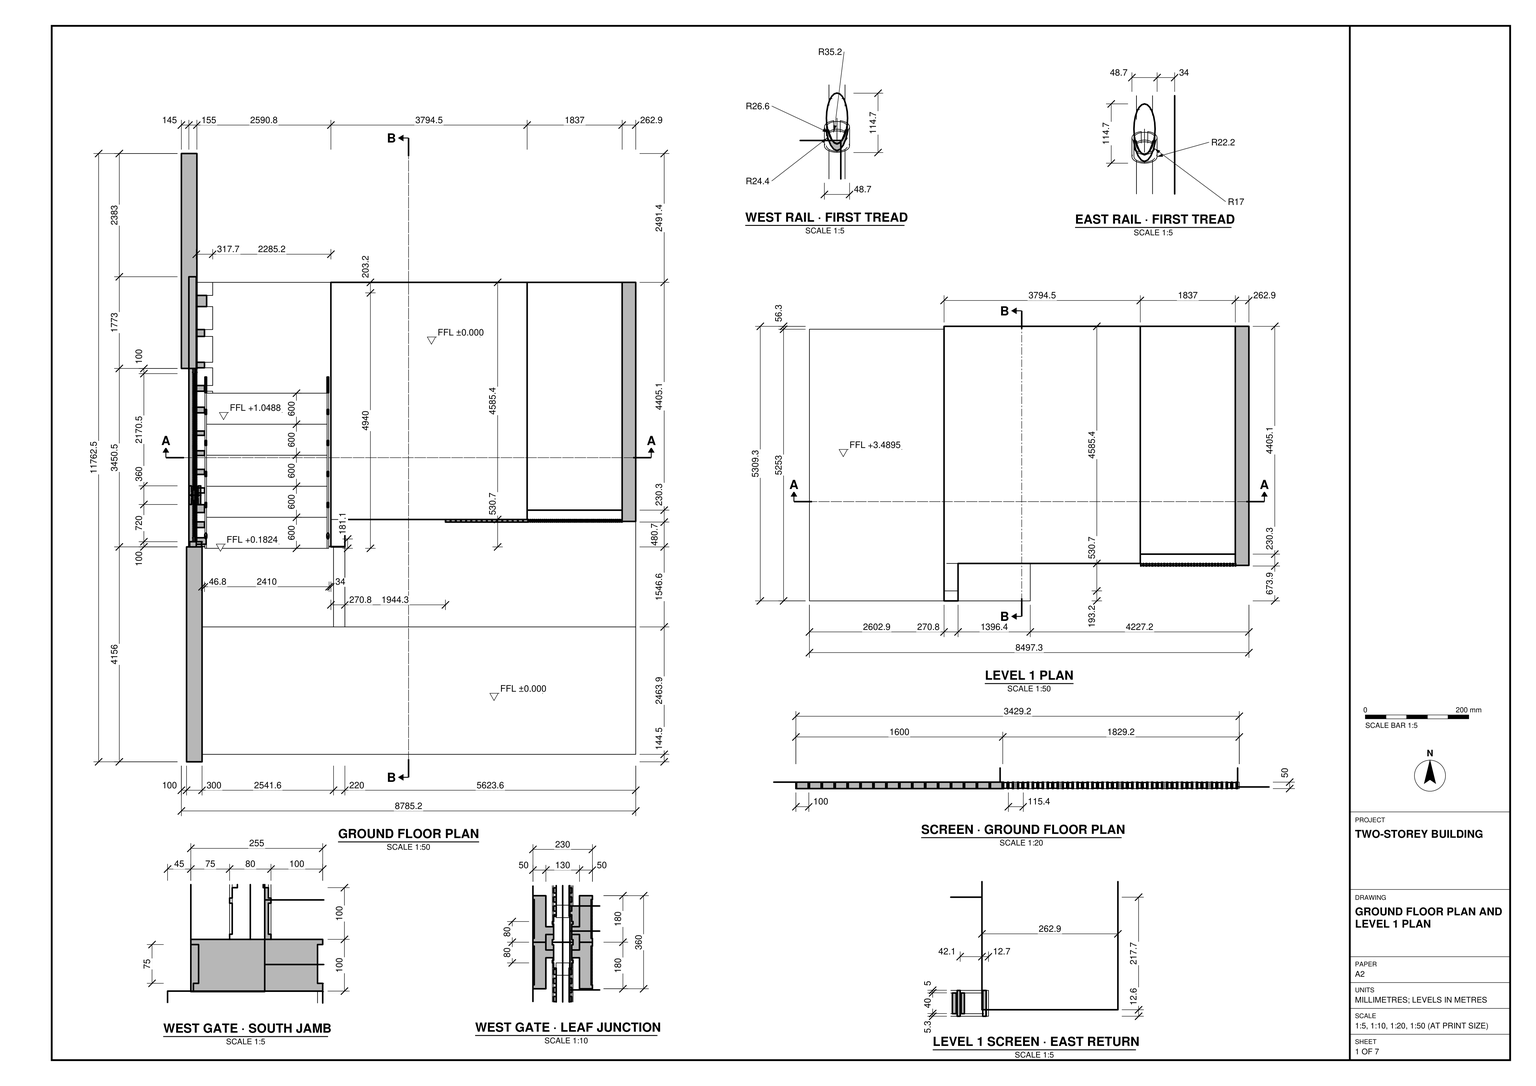
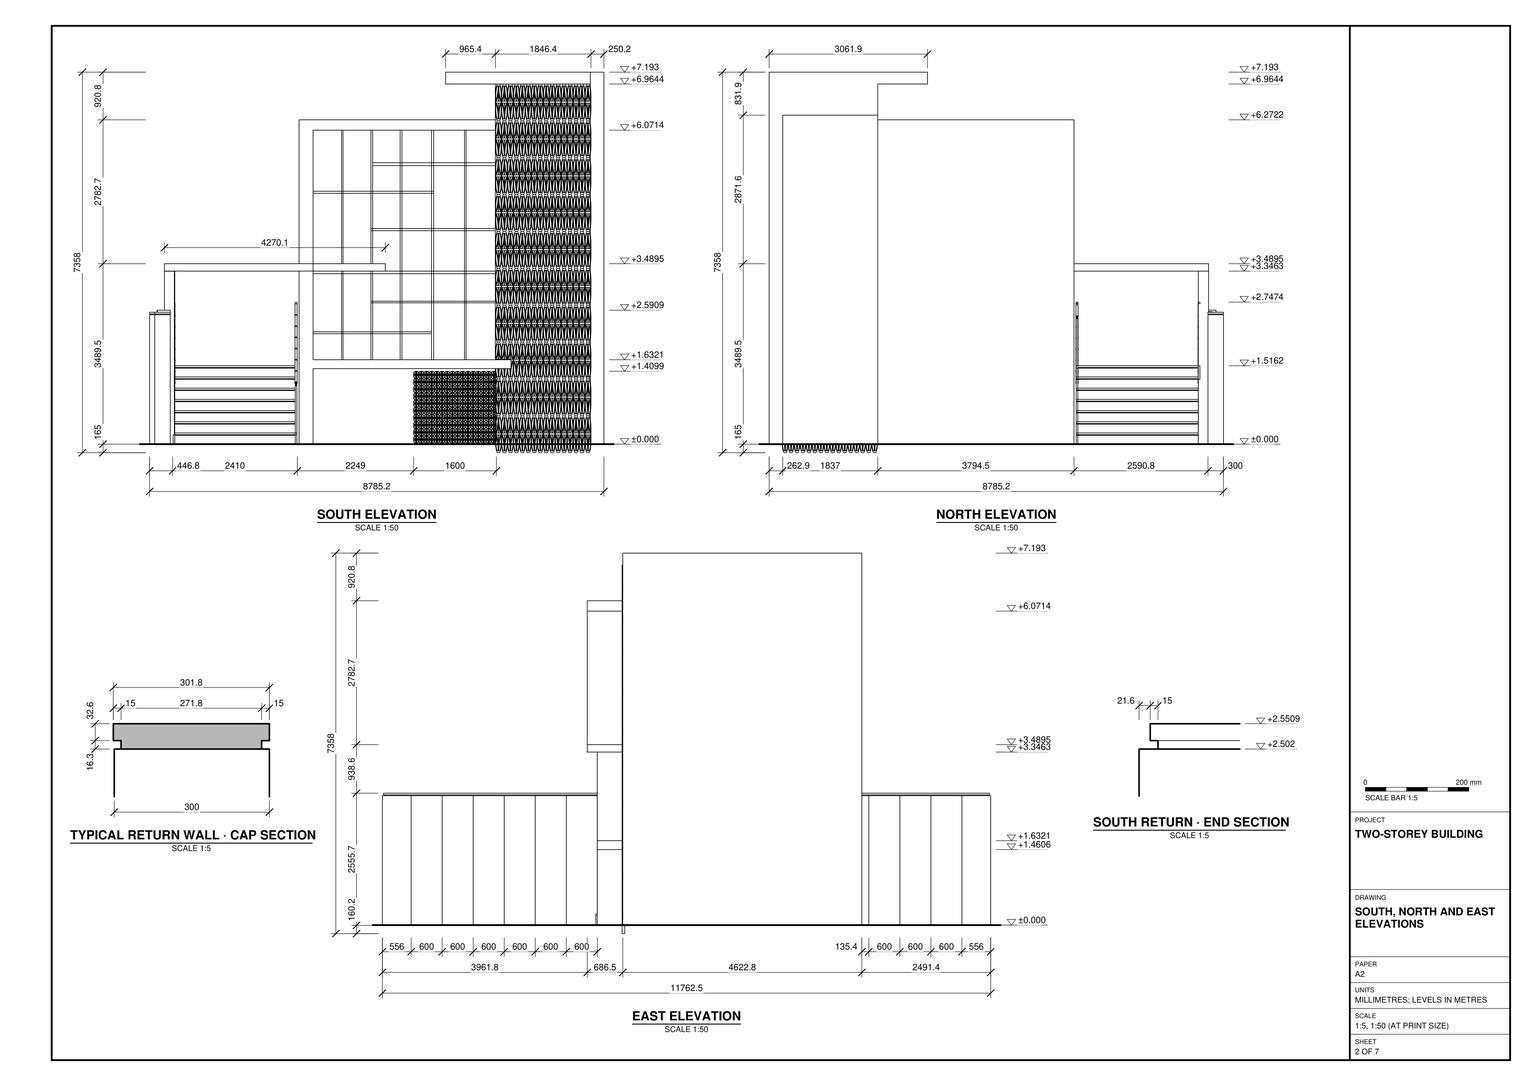
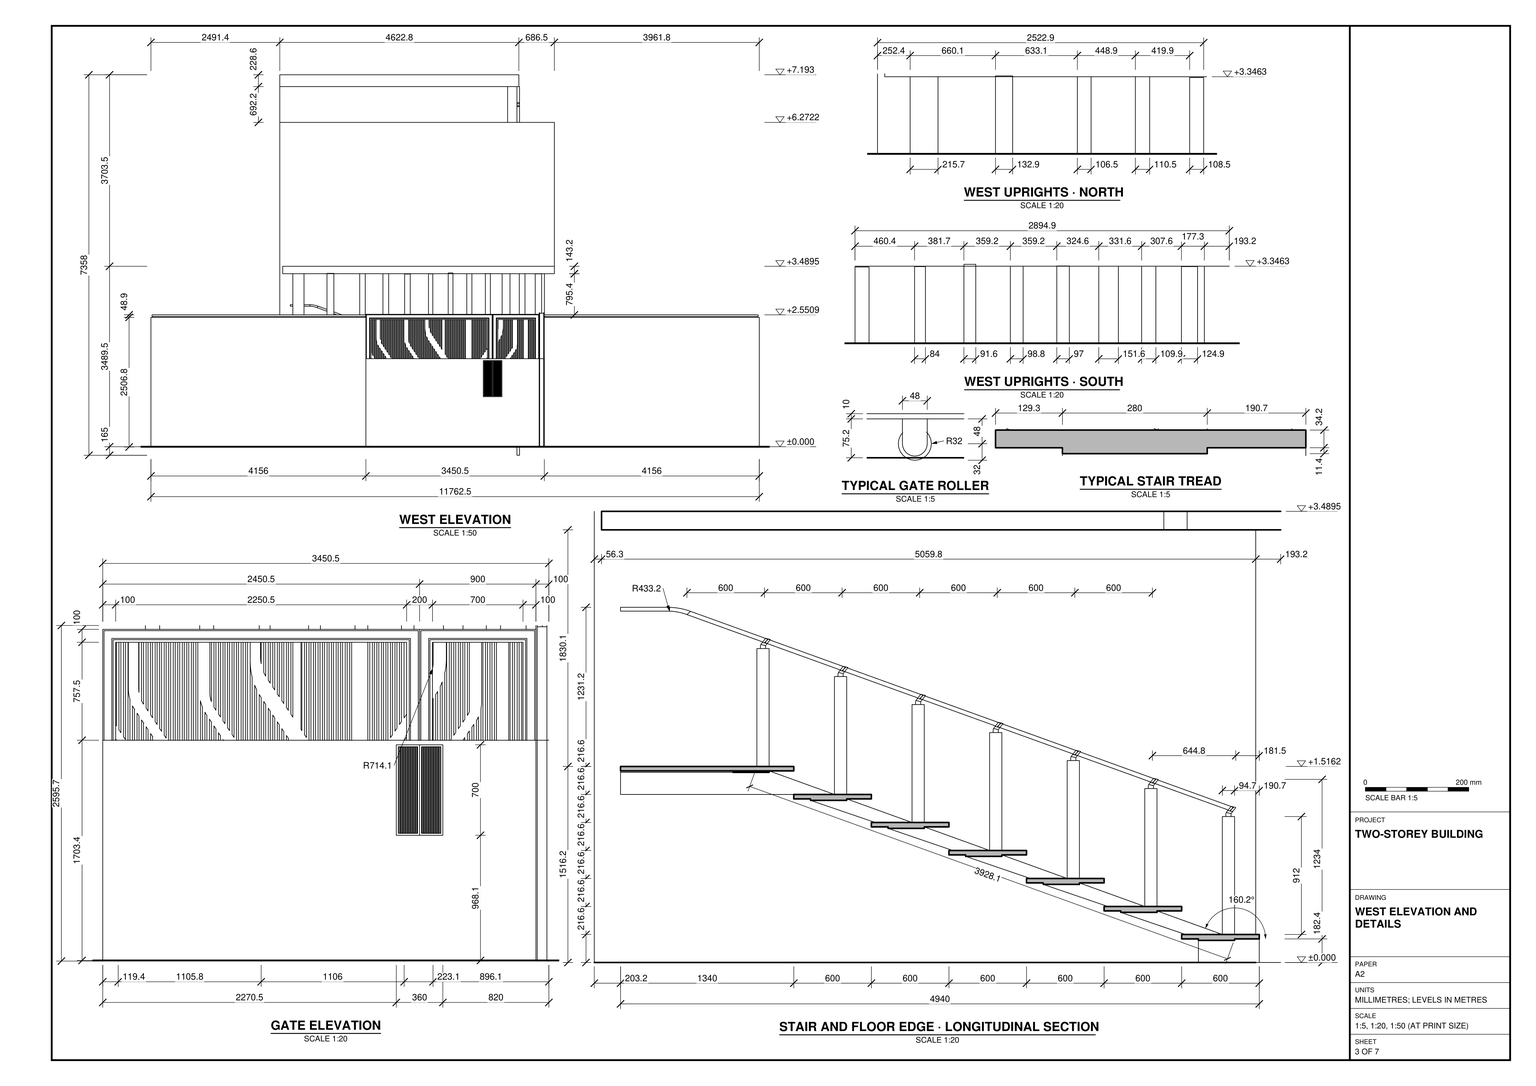
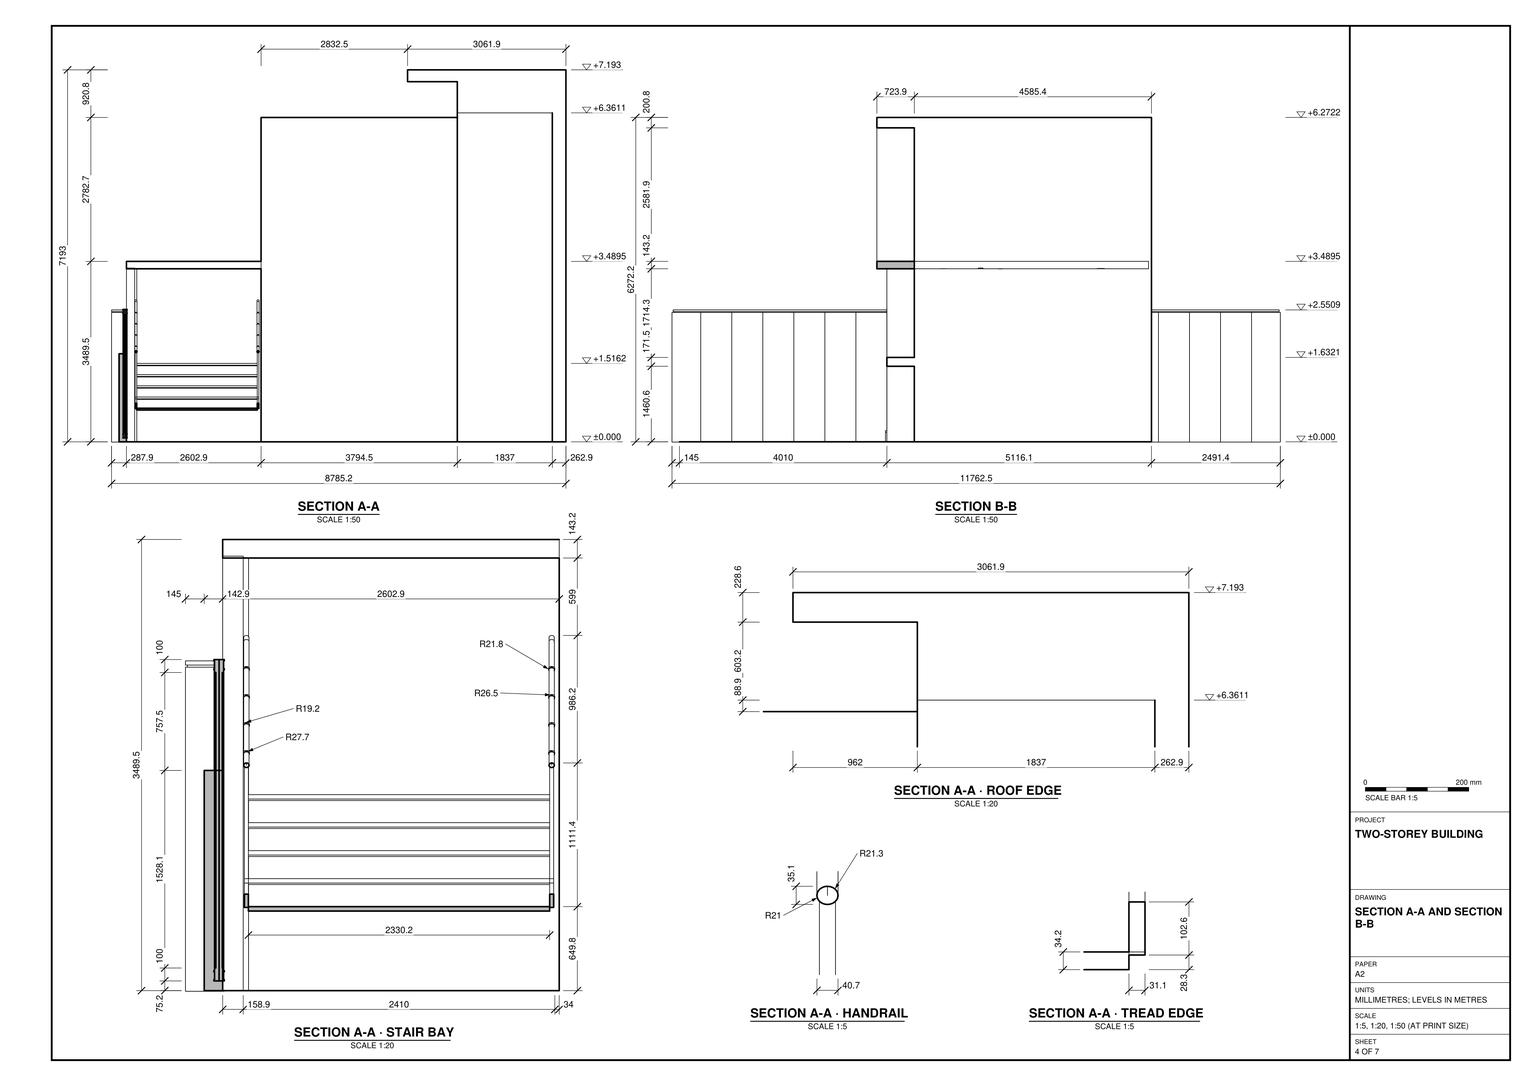
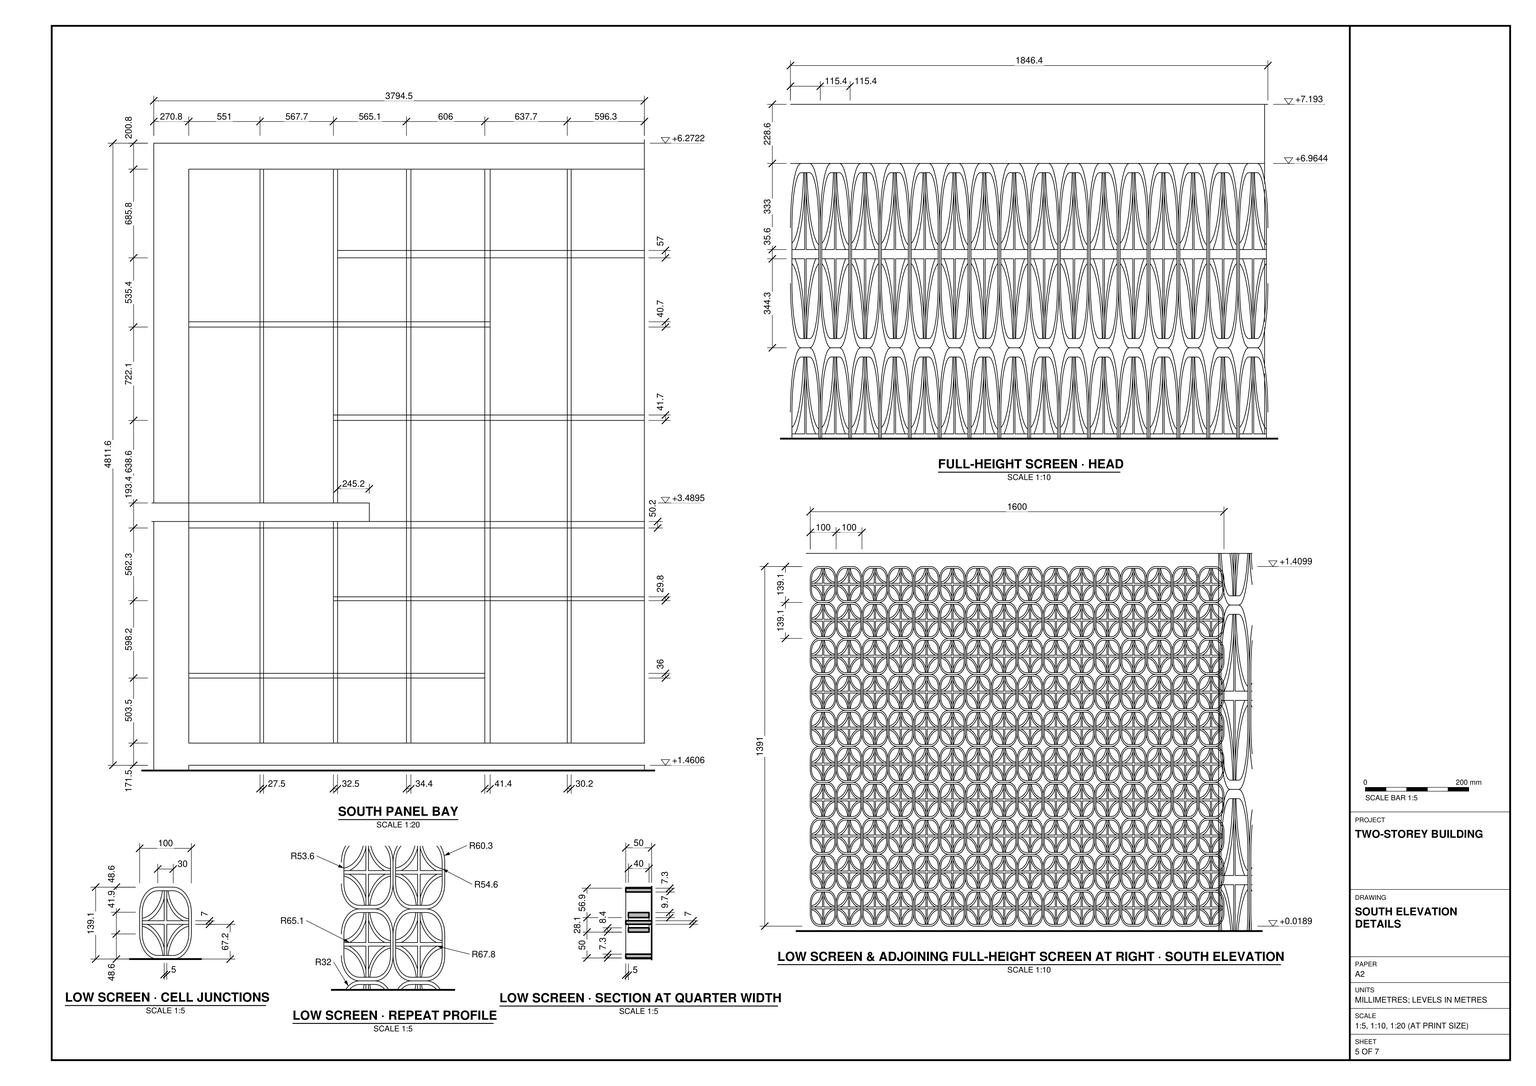
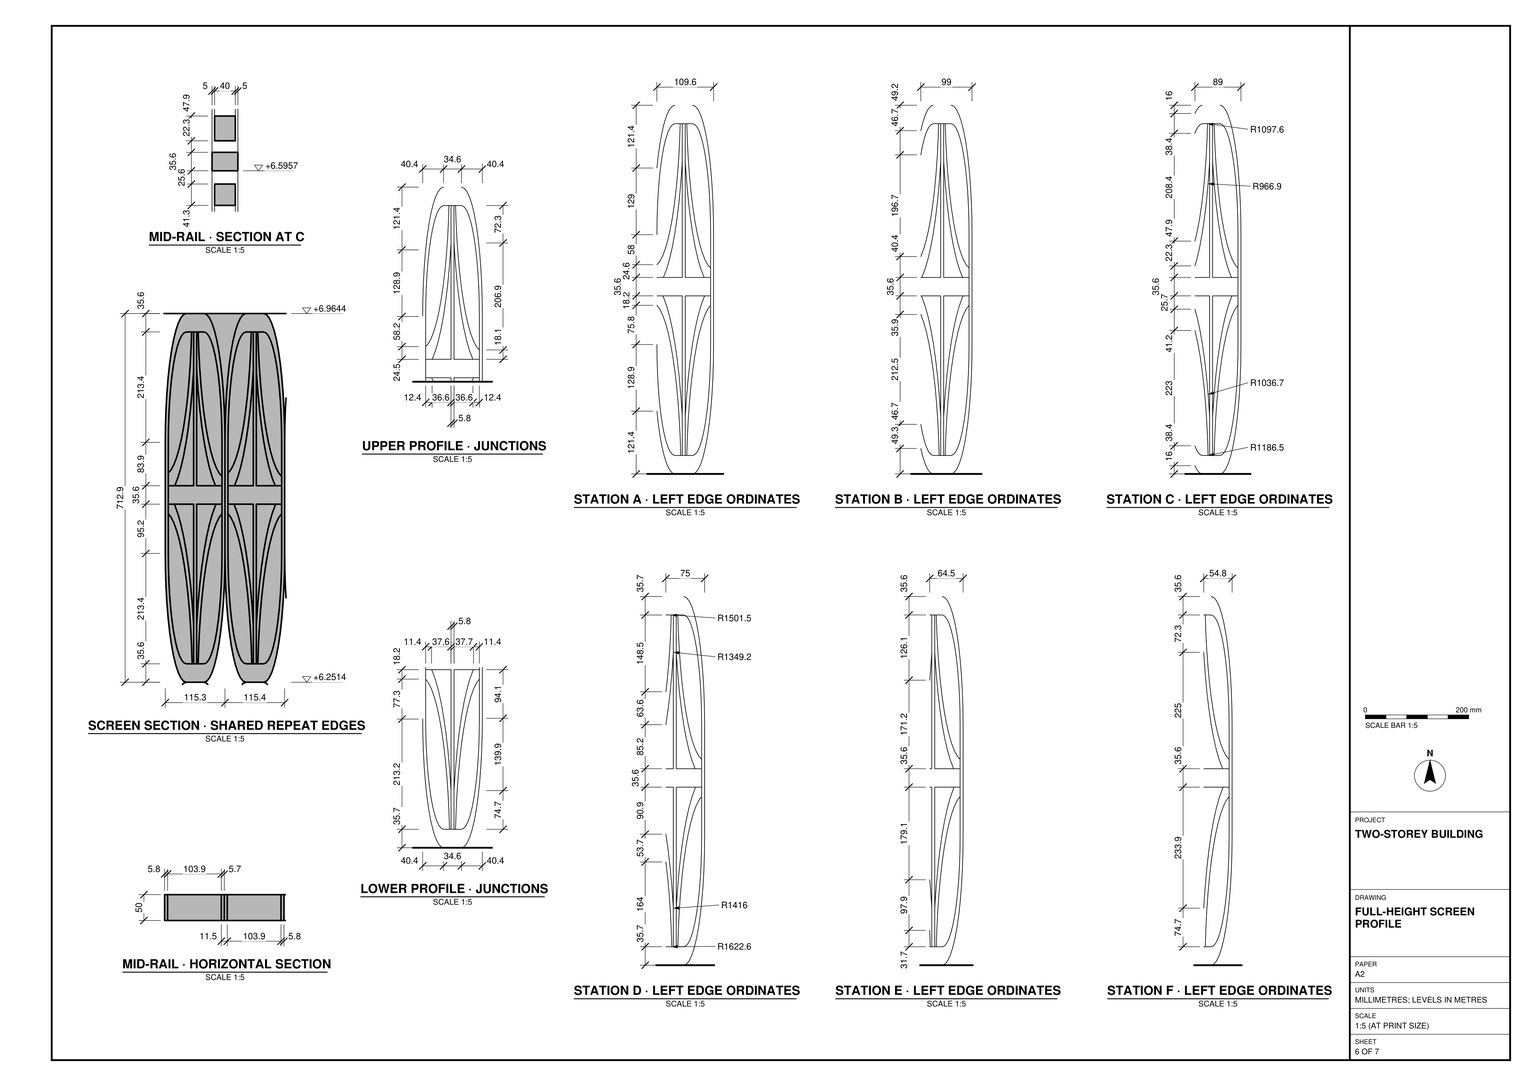
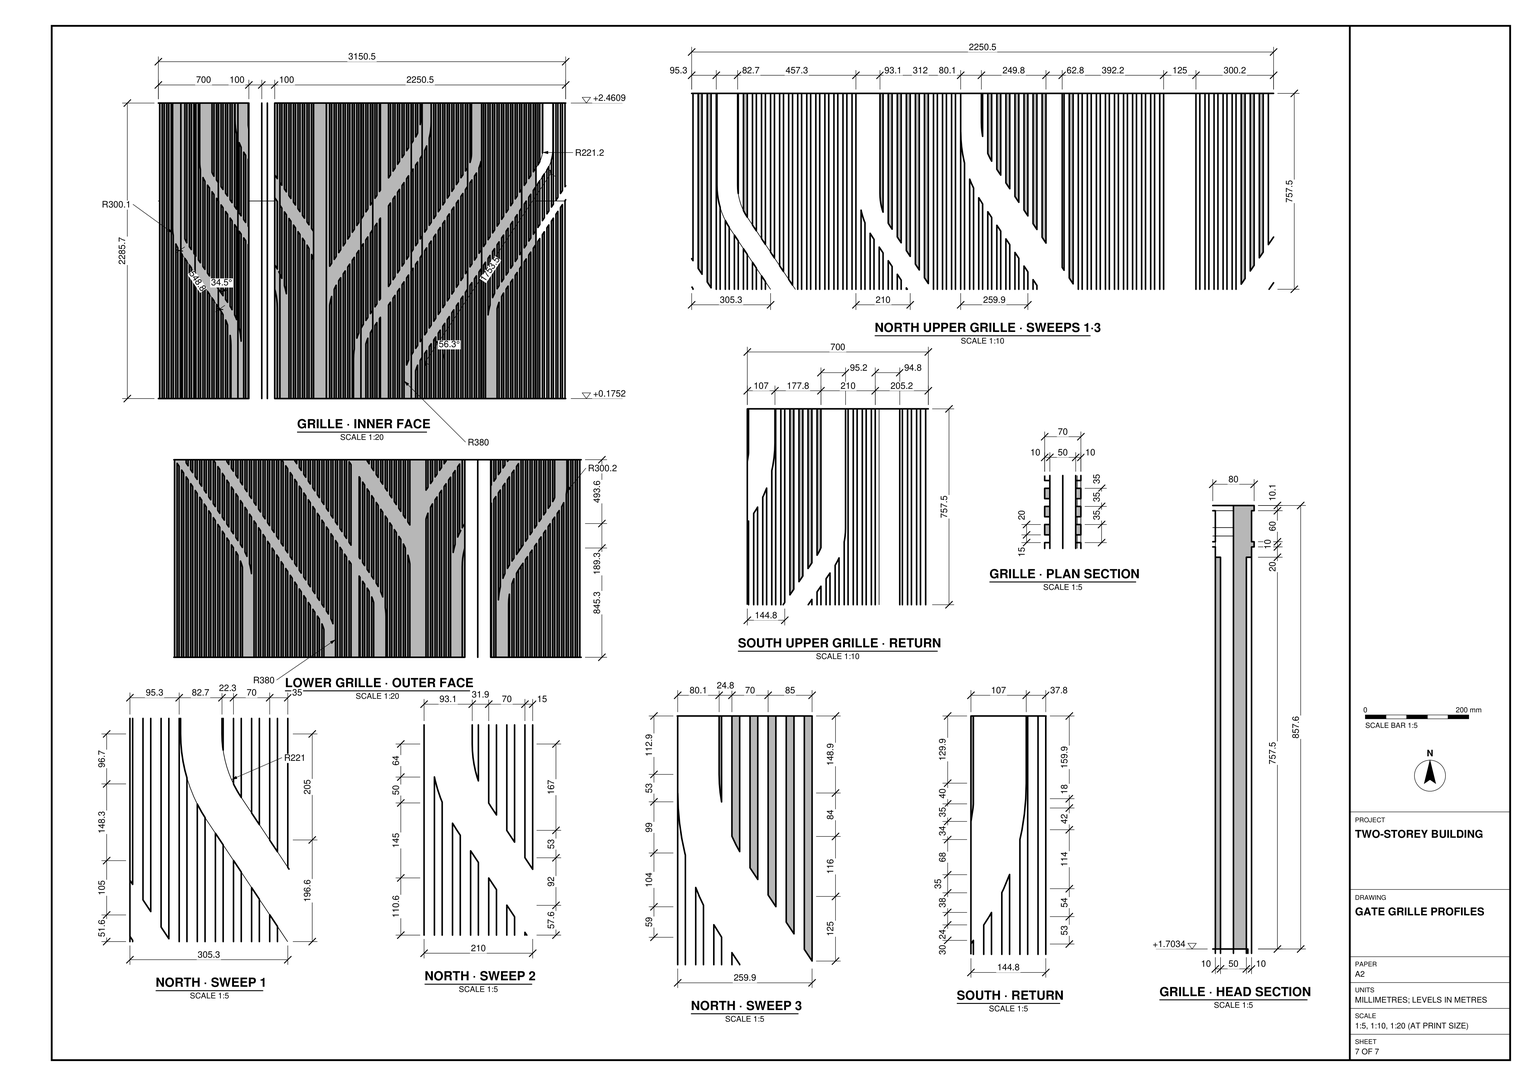
Build the two-storey building in SketchUp from task_files/diagram_01.pdf. Work in millimetres. The overall extents are 8785.2 mm east to west, 11762.5 mm north to south and 7358 mm high. Set the ground floor at 0 mm and Level 1 at +3489.5 mm.

Use the plans to lay out the floor slabs, stepped floor edges, walls and openings. Follow the wall thicknesses shown, including the 300 mm typical return walls. Match the stepped roof profile in the elevations, with the higher flat roof projecting over the tall south screen. Reproduce the framed bays on the south face, the tall diamond-pattern screen and the shorter patterned panel beside it.

Place the exterior stair along the west side. Follow the longitudinal section for the open treads, landing, sloping handrails and upright supports. Set the unequal gate leaves between the capped west boundary walls and follow the gate elevation for their solid lower panels and barred upper panels.

Keep walls, slabs, roof elements and each furniture or joinery piece shown in separate groups or components, and use components for repeated parts. Any suitable library component may be used for decor and loose items. Save one SketchUp model as output_files/two_storey_building_exterior_stair_and_screened_facade.skp.

# SketchUp Ruby script. Lengths in millimetres.
U = 1.mm
M = Sketchup.active_model
def pt(a) = Geom::Point3d.new(a.map { |v| v * U })
def face(e, loops, mat)
  f = e.add_face(loops[0].map { |a| pt(a) })
  loops[1..].each { |l| e.add_face(l.map { |a| pt(a) }).erase! }
  f.material = f.back_material = mat if mat
  f
end
# faces: each face lists its corners as indices into pts; further lists are holes
def faces(e, pts, list, mat = nil) = list.each { |f| face(e, (f[0].is_a?(Array) ? f : [f]).map { |l| l.map { |i| pts[i] } }, mat) }
# xy, xz, yz: faces in a plane at the given z, y or x. An outline is a flat list of corners, or four numbers for a rectangle; further outlines are holes
def ring(l) = l.size == 4 ? [[l[0], l[1]], [l[2], l[1]], [l[2], l[3]], [l[0], l[3]]] : l.each_slice(2).to_a
def flat(e, list, mat, &to3) = list.each { |f| face(e, (f[0].is_a?(Array) ? f : [f]).map { |l| ring(l).map { |u, v| to3.(u, v) } }, mat) }
def xy(e, z, list, mat = nil) = flat(e, list, mat) { |x, y| [x, y, z] }
def xz(e, y, list, mat = nil) = flat(e, list, mat) { |x, z| [x, y, z] }
def yz(e, x, list, mat = nil) = flat(e, list, mat) { |y, z| [x, y, z] }
def lines(e, pts, list) = list.each { |a, b| e.add_line(pt(pts[a]), pt(pts[b])) }
# prism: a flat outline (further loops are holes) pulled along v
def prism(e, loops, v, mat = nil)
  f = face(e, loops, mat); d = Geom::Vector3d.new(v.map { |x| x * U })
  f.pushpull(f.normal.samedirection?(d) ? d.length : -d.length)
end
def box(e, o, s, mat = nil) = prism(e, [[o, [o[0] + s[0], o[1], o[2]], [o[0] + s[0], o[1] + s[1], o[2]], [o[0], o[1] + s[1], o[2]]]], [0, 0, s[2]], mat)
def at(x, y, z, deg = 0) = Geom::Transformation.translation(pt([x, y, z])) * Geom::Transformation.rotation(ORIGIN, Z_AXIS, deg.degrees)
def axes(o, x, y, z) = Geom::Transformation.new([*x, 0, *y, 0, *z, 0, *pt(o).to_a, 1])
def part(name) = M.definitions.add(name)
# library, detail: a bought-in or finely detailed component or shape, given as its bounding box
def library(name, o, s) = part(name).tap { |d| box(d.entities, o, s) }
def detail(e, o, s) = box(e.add_group.entities, o, s)
def put(e, d, t, mat = nil) = e.add_instance(d, t).tap { |i| i.material = mat if mat }
def group(e, t, mat = nil) = e.add_group.tap { |g| g.transformation = t; g.material = mat if mat }.entities
root = M.entities
M.materials.add("0-370-55720370副本4").color = [155, 133, 94]
M.materials.add("Niraj_Shoe_Stitching").color = [181, 137, 92]
M.materials.add("[Asphalt New]").color = [67, 60, 62]
M.materials.add("[Metal Corrugated Shiny]16").color = [144, 125, 78]
M.materials.add("[Polished Concrete New]").color = [200, 200, 203]
M.materials.add("[Translucent Glass Gray]").color = [128, 128, 128]
M.materials["[Translucent Glass Gray]"].alpha = 0.5
M.materials.add("[Translucent_Glass_Gold]").color = [255, 219, 196]
M.materials["[Translucent_Glass_Gold]"].alpha = 0.4
M.materials.add("[Wood Cherry Original]").color = [152, 86, 42]
M.materials.add("[Wood Floor Parquet]").color = [145, 89, 39]
M.materials.add("news-2011071812072216631663").color = [231, 218, 195]
M.materials.add("主石材1").color = [201, 201, 201]
M.materials.add("材质25").color = [247, 244, 232]
c1 = library("Screened entrance gate",[5,-2322.7,-50],[255,3450.5,2595.7])
c2 = part("组\#15")
xy(c2.entities,-5,[[2833.2,0,6967.6,301.8]],"0-370-55720370副本4")
xy(c2.entities,25,[[[2833.2,0,6967.6,301.8],[2848.2,15,6952.6,286.8]]],"0-370-55720370副本4")
xy(c2.entities,40,[[2848.2,15,6952.6,286.8]],"0-370-55720370副本4")
xz(c2.entities,0,[[2833.2,-5,6967.6,25]],"0-370-55720370副本4")
xz(c2.entities,15,[[2848.2,25,6952.6,40]],"0-370-55720370副本4")
xz(c2.entities,286.8,[[2848.2,25,6952.6,40]],"0-370-55720370副本4")
xz(c2.entities,301.8,[[2833.2,-5,6967.6,25]],"0-370-55720370副本4")
yz(c2.entities,2833.2,[[0,-5,301.8,25]],"0-370-55720370副本4")
yz(c2.entities,2848.2,[[15,25,286.8,40]],"0-370-55720370副本4")
yz(c2.entities,6952.6,[[15,25,286.8,40]],"0-370-55720370副本4")
yz(c2.entities,6967.6,[[0,-5,301.8,25]],"0-370-55720370副本4")
c3 = part("组\#14")
xy(c3.entities,400,[[10,-30,160,20]],"[Metal Corrugated Shiny]16")
xy(c3.entities,410,[[0,-30,170,20]],"[Metal Corrugated Shiny]16")
xz(c3.entities,-30,[[0,0,10,0,10,400,160,400,160,0,170,0,170,410,0,410]],"[Metal Corrugated Shiny]16")
xz(c3.entities,20,[[10,400,0,410,170,410,160,400]],"[Metal Corrugated Shiny]16")
yz(c3.entities,0,[[-30,0,-30,410,20,410]],"[Metal Corrugated Shiny]16")
yz(c3.entities,10,[[-30,0,20,400,-30,400]],"[Metal Corrugated Shiny]16")
yz(c3.entities,160,[[-30,0,-30,400,20,400]],"[Metal Corrugated Shiny]16")
yz(c3.entities,170,[[-30,0,20,410,-30,410]],"[Metal Corrugated Shiny]16")
p = [[10,-5,200],[0,-5,205],[0,-30,0],[10,-30,0],[170,-5,205],[160,-5,200],
  [170,-30,0],[160,-30,0],[10,20,400],[160,20,400],[0,20,410],[170,20,410]]
faces(c3.entities,p,[[0,1,2],[0,2,3],[4,5,6],[6,5,7],[8,1,0],[4,9,5],[8,10,1],[11,9,4]],"[Metal Corrugated Shiny]16")
c4 = part("组\#1730")
xy(c4.entities,498.2,[[-300,0,3856,300]],"主石材1")
xy(c4.entities,2153.5,[[3483.5,250,3633.5,300]],"[Metal Corrugated Shiny]16")
xy(c4.entities,2803.2,[[-300,0,3856,300]],"主石材1")
xz(c4.entities,0,[[-300,498.2,3856,2803.2]],"主石材1")
xz(c4.entities,300,[[[-300,498.2,3856,2803.2],[3473.5,1753.5,3643.5,2163.5]],[3473.5,1753.5,3473.5,2163.5,3643.5,2163.5,3643.5,1753.5,3633.5,1753.5,3633.5,2153.5,3483.5,2153.5,3483.5,1753.5]],"主石材1")
yz(c4.entities,-300,[[0,498.2,300,2803.2]],"主石材1")
yz(c4.entities,3483.5,[[300,1753.5,300,2153.5,250,2153.5]],"[Metal Corrugated Shiny]16")
yz(c4.entities,3633.5,[[300,1753.5,250,2153.5,300,2153.5]],"[Metal Corrugated Shiny]16")
yz(c4.entities,3856,[[0,498.2,300,2803.2]],"主石材1")
p = [[3483.5,250,2153.5],[3633.5,250,2153.5],[3633.5,300,1753.5],[3483.5,300,1753.5],[3613.5,252.5,2133.6],[3503.5,252.5,2133.6],
  [3503.5,297.5,1773.3],[3613.5,297.5,1773.3],[3608.9,272.5,1973.8],[3508.2,272.5,1973.8],[3508.2,273,1969.7],[3508.2,296.9,1778],
  [3608.9,296.9,1778],[3608.9,273,1969.7],[3608.9,253.1,2129],[3508.2,253.1,2129],[3548.5,255.1,2112.9],[3548.5,257.2,2096.3],
  [3567.4,257.2,2096.3],[3567.4,255.1,2112.9],[3548.5,262.3,2055.4],[3548.5,264.3,2038.7],[3567.4,264.3,2038.7],[3567.4,262.3,2055.4],
  [3518,265.9,2026.6],[3518,267.9,2009.9],[3536.9,267.9,2009.9],[3536.9,265.9,2026.6],[3579,265.9,2026.6],[3579,267.9,2009.9],
  [3597.9,267.9,2009.9],[3597.9,265.9,2026.6],[3518,258.7,2084.2],[3518,260.7,2067.5],[3536.9,260.7,2067.5],[3536.9,258.7,2084.2],
  [3579,262.3,2055.4],[3579,264.3,2038.7],[3597.9,264.3,2038.7],[3597.9,262.3,2055.4],[3579,258.7,2084.2],[3579,260.7,2067.5],
  [3597.9,260.7,2067.5],[3597.9,258.7,2084.2],[3518,262.3,2055.4],[3518,264.3,2038.7],[3536.9,264.3,2038.7],[3536.9,262.3,2055.4],
  [3518,255.1,2112.9],[3518,257.2,2096.3],[3536.9,257.2,2096.3],[3536.9,255.1,2112.9],[3548.5,265.9,2026.6],[3548.5,267.9,2009.9],
  [3567.4,267.9,2009.9],[3567.4,265.9,2026.6],[3579,255.1,2112.9],[3579,257.2,2096.3],[3597.9,257.2,2096.3],[3597.9,255.1,2112.9],
  [3548.5,258.7,2084.2],[3548.5,260.7,2067.5],[3567.4,260.7,2067.5],[3567.4,258.7,2084.2]]
faces(c4.entities,p,[[[0,1,2,3],[4,5,6,7]],[[5,4,7,6],[8,9,10,11,12,13]],[10,13,12,11],[13,10,9,8],[[14,8,9,15],[16,17,18,19],[20,21,22,23],[24,25,26,27],[28,29,30,31],[32,33,34,35],[36,37,38,39],[40,41,42,43],[44,45,46,47],[48,49,50,51],[52,53,54,55],[56,57,58,59],[60,61,62,63]],[25,24,27,26],[53,52,55,54],[29,28,31,30],
  [45,44,47,46],[21,20,23,22],[37,36,39,38],[33,32,35,34],[61,60,63,62],[41,40,43,42],[49,48,51,50],[17,16,19,18],
  [57,56,59,58]],"[Metal Corrugated Shiny]16")
put(c4.entities,c3,at(3473.5,330,1753.5))
c5 = part("组\#263")
p = [[3856,300,498.2],[3856,300,2803.2],[3256,300,498.2],[3256,300,2803.2],[2656,300,498.2],[2656,300,2803.2],
  [2056,300,498.2],[2056,300,2803.2],[1456,300,498.2],[1456,300,2803.2],[856,300,498.2],[856,300,2803.2],
  [256,300,498.2],[256,300,2803.2]]
lines(c5.entities,p,[[0,1],[0,2],[2,3],[4,5],[6,7],[8,9],[10,11],[12,13],[10,12],[8,10],[6,8],[4,6],
  [2,4]])
put(c5.entities,c2,axes([6689.2,0,2843.2],[-1,0,0],[0,1,0],[0,0,-1]))
put(c5.entities,c4,at(0,0,0))
c6 = part("组\#1715")
xy(c6.entities,-5,[[2833.2,0,6967.6,301.8]],"0-370-55720370副本4")
xy(c6.entities,25,[[[2833.2,0,6967.6,301.8],[2848.2,15,6952.6,286.8]]],"0-370-55720370副本4")
xy(c6.entities,40,[[2848.2,15,6952.6,286.8]],"0-370-55720370副本4")
xz(c6.entities,0,[[2833.2,-5,6967.6,25]],"0-370-55720370副本4")
xz(c6.entities,15,[[2848.2,25,6952.6,40]],"0-370-55720370副本4")
xz(c6.entities,286.8,[[2848.2,25,6952.6,40]],"0-370-55720370副本4")
xz(c6.entities,301.8,[[2833.2,-5,6967.6,25]],"0-370-55720370副本4")
yz(c6.entities,2833.2,[[0,-5,301.8,25]],"0-370-55720370副本4")
yz(c6.entities,2848.2,[[15,25,286.8,40]],"0-370-55720370副本4")
yz(c6.entities,6952.6,[[15,25,286.8,40]],"0-370-55720370副本4")
yz(c6.entities,6967.6,[[0,-5,301.8,25]],"0-370-55720370副本4")
c7 = part("组\#17")
box(c7.entities,[-300,0,498.2],[4156,300,2305],"主石材1")
c8 = part("组\#18")
p = [[3856,300,498.2],[3856,300,2803.2],[3256,300,498.2],[3256,300,2803.2],[2656,300,498.2],[2656,300,2803.2],
  [2056,300,498.2],[2056,300,2803.2],[1456,300,498.2],[1456,300,2803.2],[856,300,498.2],[856,300,2803.2],
  [256,300,498.2],[256,300,2803.2]]
lines(c8.entities,p,[[0,1],[0,2],[2,3],[4,5],[6,7],[8,9],[10,11],[12,13],[10,12],[8,10],[6,8],[4,6],
  [2,4]])
put(c8.entities,c6,axes([6689.2,0,2843.2],[-1,0,0],[0,1,0],[0,0,-1]))
put(c8.entities,c7,at(0,0,0))
c9 = part("CỔNG+3+(4)")
put(c9.entities,c1,at(-5,2323.7,45.2))
put(c9.entities,c5,axes([-145,7307.5,-546.5],[0,-1,0],[1,0,0],[0,0,1.08753]))
put(c9.entities,c8,axes([-45,-3855,-546.5],[0,1,0],[1,0,0],[0,0,1.08753]))
c10 = library("MINJANE_01_窗花",[-456.2,3539.8,0],[3200,50,2000])
c11 = library("Trappe+færdig",[-6469.8,1752.5,0],[2410,4940,2747.4])
xy(root,0,[[145,4155,287.9,9379.5],[287.9,4155,605.6,4207.4],[2890.8,4155,3161.6,4685.7],[287.9,4332.3,605.6,4530],[287.9,4639.9,605.6,4819.9],
  [8522.3,4648.3,8785.2,9271.1],[2890.8,4685.7,6685.3,9271.1],[6685.3,4865.9,8522.3,9271.1],[287.9,4971.5,605.6,5199.1],[287.9,5296.1,605.6,5556.6],
  [287.9,5655.4,605.6,5922.9],[287.9,6014.5,605.6,6312.2],[287.9,6396.2,605.6,6748.2],[287.9,6856.7,605.6,7166.1],[287.9,7276.6,605.6,7619],
  [287.9,7725.5,605.6,8225.7],[287.9,8358.6,605.6,8802.9],[287.9,9018.7,605.6,9271.1]])
xy(root,0,[[400,144.5,8785.2,2608.4],[2941.6,2608.4,8785.2,2608.4,8785.2,4648.3,8522.3,4648.3,8522.3,4865.9,6685.3,4865.9,6685.3,4685.7,3161.6,4685.7,3161.6,4155,2941.6,4155],[605.6,4155,605.6,4207.4,478.6,4207.4,478.6,4332.3,605.6,4332.3,605.6,4530,446.8,4530,446.8,4639.9,605.6,4639.9,605.6,4819.9,446.8,4819.9,446.8,4971.5,605.6,4971.5,605.6,5199.1,446.8,5199.1,446.8,5296.1,605.6,5296.1,605.6,5556.6,446.8,5556.6,446.8,5655.4,605.6,5655.4,605.6,5922.9,446.8,5922.9,446.8,6014.5,605.6,6014.5,605.6,6312.2,446.8,6312.2,446.8,6396.2,605.6,6396.2,605.6,6748.2,446.8,6748.2,446.8,6856.7,605.6,6856.7,605.6,7166.1,446.8,7166.1,446.8,7276.6,605.6,7276.6,605.6,7619,446.8,7619,446.8,7725.5,605.6,7725.5,605.6,8225.7,446.8,8225.7,446.8,8358.6,605.6,8358.6,605.6,8802.9,488.1,8802.9,488.1,9018.7,605.6,9018.7,605.6,9271.1,2890.8,9271.1,2890.8,4155]],"[Polished Concrete New]")
xy(root,1460.6,[[3161.6,4155,6988.5,4685.7]])
xy(root,1632.1,[[3161.6,4155,6988.5,4685.7]])
xy(root,1703.4,[[145,4155,287.9,9379.5]])
xy(root,3340.1,[[287.9,6748.2,446.8,6856.7]])
xy(root,3343.3,[[287.9,6312.2,446.8,6396.2]])
xy(root,3343.4,[[287.9,4207.4,478.6,4332.3]])
xy(root,3346.3,[[287.9,3961.8,287.9,4530,446.8,4530,446.8,4639.9,287.9,4639.9,287.9,4819.9,446.8,4819.9,446.8,4971.5,287.9,4971.5,287.9,5556.6,446.8,5556.6,446.8,5655.4,287.9,5655.4,287.9,7619,446.8,7619,446.8,7725.5,287.9,7725.5,287.9,8802.9,488.1,8802.9,488.1,9018.7,605.6,9018.7,605.6,9214.8,2890.8,9214.8,2890.8,3961.8],[2890.8,3961.8,3161.6,4155],[3161.6,3961.8,4558,4685.7],[287.9,8802.9,488.1,9018.7],[287.9,9018.7,605.6,9214.8]])
xy(root,3346.4,[[287.9,7166.1,446.8,7276.6]])
xy(root,3348,[[287.9,5199.1,446.8,5296.1]])
xy(root,3352.8,[[287.9,8225.7,446.8,8358.6]])
xy(root,3360.7,[[287.9,5922.9,446.8,6014.5]])
xy(root,3489.5,[[287.9,3961.8,2890.8,9214.8],[3161.6,3961.8,4558,4685.7]],"[Wood Cherry Original]")
xy(root,6071.4,[[3161.6,3961.8,6685.3,4685.7]])
xy(root,6272.2,[[2890.8,3961.8,6685.3,9271.1]],"材质25")
xy(root,6964.4,[[5723.3,4648.3,5723.3,9271.1,6685.3,9271.1,6685.3,4865.9,8522.3,4865.9,8522.3,4648.3]])
xy(root,7193,[[5723.3,4648.3,8785.2,9271.1]],"材质25")
xz(root,3961.8,[[3161.6,3346.3,4558,3489.5]],"[Wood Cherry Original]")
xz(root,3961.8,[[287.9,3346.3,3161.6,3489.5]],"[Wood Floor Parquet]")
xz(root,3961.8,[[2890.8,3489.5,3161.6,3489.5,3161.6,6071.4,6685.3,6071.4,6685.3,6272.2,2890.8,6272.2]],"材质25")
xz(root,4155,[[145,0,287.9,1703.4]])
xz(root,4155,[[2890.8,0,3161.6,0,3161.6,1460.6,6988.5,1460.6,6988.5,1632.1,3161.6,1632.1,3161.6,3346.3,2890.8,3346.3]],"材质25")
xz(root,4207.4,[[287.9,0,478.6,3343.4]],"[Wood Floor Parquet]")
xz(root,4332.3,[[287.9,0,478.6,3343.4]])
xz(root,4530,[[287.9,0,446.8,3346.3]],"[Wood Floor Parquet]")
xz(root,4639.9,[[287.9,0,446.8,3346.3]])
xz(root,4648.3,[[8522.3,0,8785.2,7193],[5723.3,6964.4,8522.3,7193]],"材质25")
xz(root,4685.7,[[6685.3,1460.6,6988.5,1632.1],[3712.6,3346.3,3740.1,3489.5],[3740.1,3346.3,3838.4,3489.5],[3838.4,3346.3,3859.8,3489.5],[3859.8,3346.3,4280.3,3489.5],
  [4280.3,3346.3,4312.8,3489.5],[4312.8,3346.3,4542.1,3489.5],[4542.1,3346.3,4558,3489.5]])
xz(root,4685.7,[[3712.6,1632.1,3740.1,2135.6],[4280.3,1632.1,4312.8,2135.6],[4845.4,1632.1,4879.8,2135.6],[5451.3,1632.1,5492.7,2733.8],[6089,1632.1,6119.2,2733.8],
  [3161.6,2135.6,3712.6,2171.5],[3712.6,2135.6,3740.1,2171.5],[3740.1,2135.6,4280.3,2171.5],[4280.3,2135.6,4312.8,2171.5],[4312.8,2135.6,4845.4,2171.5],
  [4845.4,2135.6,4879.8,2171.5],[4879.8,2135.6,5451.3,2171.5],[3712.6,2171.5,3740.1,3296.1],[4280.3,2171.5,4312.8,2733.8],[4845.4,2171.5,4879.8,2733.8],
  [4280.3,2733.8,4312.8,2763.6],[4312.8,2733.8,4845.4,2763.6],[4845.4,2733.8,4879.8,2763.6],[4879.8,2733.8,5451.3,2763.6],[5451.3,2733.8,5492.7,2763.6],
  [5492.7,2733.8,6089,2763.6],[6089,2733.8,6119.2,2763.6],[6119.2,2733.8,6685.3,2763.6],[4280.3,2763.6,4312.8,3296.1],[4845.4,2763.6,4879.8,3296.1],
  [5451.3,2763.6,5492.7,3296.1],[6089,2763.6,6119.2,3296.1],[3161.6,3296.1,3712.6,3346.3],[3712.6,3296.1,3740.1,3346.3],[3740.1,3296.1,4280.3,3346.3],
  [4280.3,3296.1,4312.8,3346.3],[4312.8,3296.1,4845.4,3346.3],[4845.4,3296.1,4879.8,3346.3],[4879.8,3296.1,5451.3,3346.3],[5451.3,3296.1,5492.7,3346.3],
  [5492.7,3296.1,6089,3346.3],[6089,3296.1,6119.2,3346.3],[6119.2,3296.1,6685.3,3346.3],[4845.4,3346.3,4879.8,4128.1],[5451.3,3346.3,5492.7,4128.1],
  [6089,3346.3,6119.2,4128.1],[3712.6,3489.5,3740.1,4850.3],[4280.3,3489.5,4312.8,4128.1],[4280.3,4128.1,4312.8,4169.9],[4312.8,4128.1,4845.4,4169.9],
  [4845.4,4128.1,4879.8,4169.9],[4879.8,4128.1,5451.3,4169.9],[5451.3,4128.1,5492.7,4169.9],[5492.7,4128.1,6089,4169.9],[6089,4128.1,6119.2,4169.9],
  [6119.2,4128.1,6685.3,4169.9],[4280.3,4169.9,4312.8,4850.3],[4845.4,4169.9,4879.8,4850.3],[5451.3,4169.9,5492.7,4850.3],[6089,4169.9,6119.2,5385.7],
  [3161.6,4850.3,3712.6,4891],[3712.6,4850.3,3740.1,4891],[3740.1,4850.3,4280.3,4891],[4280.3,4850.3,4312.8,4891],[4312.8,4850.3,4845.4,4891],
  [4845.4,4850.3,4879.8,4891],[4879.8,4850.3,5451.3,4891],[5451.3,4850.3,5492.7,4891],[3712.6,4891,3740.1,6071.4],[4280.3,4891,4312.8,6071.4],
  [4845.4,4891,4879.8,5385.7],[5451.3,4891,5492.7,5385.7],[4312.8,5385.7,4845.4,5442.7],[4845.4,5385.7,4879.8,5442.7],[4879.8,5385.7,5451.3,5442.7],
  [5451.3,5385.7,5492.7,5442.7],[5492.7,5385.7,6089,5442.7],[6089,5385.7,6119.2,5442.7],[6119.2,5385.7,6685.3,5442.7],[4845.4,5442.7,4879.8,6071.4],
  [5451.3,5442.7,5492.7,6071.4],[6089,5442.7,6119.2,6071.4]],"[Asphalt New]")
xz(root,4685.7,[[3161.6,1632.1,3712.6,2135.6],[3740.1,1632.1,4280.3,2135.6],[4312.8,1632.1,4845.4,2135.6],[4879.8,1632.1,5451.3,2135.6],[5492.7,1632.1,6089,2733.8],
  [6119.2,1632.1,6685.3,2733.8],[3161.6,2171.5,3712.6,3296.1],[3740.1,2171.5,4280.3,3296.1],[4312.8,2171.5,4845.4,2733.8],[4879.8,2171.5,5451.3,2733.8],
  [4312.8,2763.6,4845.4,3296.1],[4879.8,2763.6,5451.3,3296.1],[5492.7,2763.6,6089,3296.1],[6119.2,2763.6,6685.3,3296.1],[4558,3346.3,4845.4,3346.3,4845.4,4128.1,4312.8,4128.1,4312.8,3489.5,4558,3489.5],
  [4879.8,3346.3,5451.3,4128.1],[5492.7,3346.3,6089,4128.1],[6119.2,3346.3,6685.3,4128.1],[3161.6,3489.5,3712.6,4850.3],[3740.1,3489.5,4280.3,4850.3],
  [4312.8,4169.9,4845.4,4850.3],[4879.8,4169.9,5451.3,4850.3],[5492.7,4169.9,6089,5385.7],[6119.2,4169.9,6685.3,5385.7],[3161.6,4891,3712.6,6071.4],
  [3740.1,4891,4280.3,6071.4],[4312.8,4891,4845.4,5385.7],[4879.8,4891,5451.3,5385.7],[4312.8,5442.7,4845.4,6071.4],[4879.8,5442.7,5451.3,6071.4],
  [5492.7,5442.7,6089,6071.4],[6119.2,5442.7,6685.3,6071.4]],"[Translucent Glass Gray]")
xz(root,4685.7,[[3161.6,0,6685.3,1460.6]],"[Translucent_Glass_Gold]")
xz(root,4819.9,[[287.9,0,446.8,3346.3]],"[Wood Floor Parquet]")
xz(root,4865.9,[[6685.3,0,8522.3,6964.4]])
xz(root,4971.5,[[287.9,0,446.8,3346.3]])
xz(root,5199.1,[[287.9,0,446.8,3348]],"[Wood Floor Parquet]")
xz(root,5296.1,[[287.9,0,446.8,3348]])
xz(root,5556.6,[[287.9,0,446.8,3346.3]],"[Wood Floor Parquet]")
xz(root,5655.4,[[287.9,0,446.8,3346.3]])
xz(root,5922.9,[[287.9,0,446.8,3360.7]],"[Wood Floor Parquet]")
xz(root,6014.5,[[287.9,0,446.8,3360.7]])
xz(root,6312.2,[[287.9,0,446.8,3343.3]],"[Wood Floor Parquet]")
xz(root,6396.2,[[287.9,0,446.8,3343.3]])
xz(root,6748.2,[[287.9,0,446.8,3340.1]],"[Wood Floor Parquet]")
xz(root,6856.7,[[287.9,0,446.8,3340.1]])
xz(root,7166.1,[[287.9,0,446.8,3346.4]],"[Wood Floor Parquet]")
xz(root,7276.6,[[287.9,0,446.8,3346.4]])
xz(root,7619,[[287.9,0,446.8,3346.3]],"[Wood Floor Parquet]")
xz(root,7725.5,[[287.9,0,446.8,3346.3]])
xz(root,8225.7,[[287.9,0,446.8,3352.8]],"[Wood Floor Parquet]")
xz(root,8358.6,[[287.9,0,446.8,3352.8]])
xz(root,8802.9,[[287.9,0,488.1,3346.3]],"[Wood Floor Parquet]")
xz(root,9018.7,[[287.9,0,488.1,3346.3]])
xz(root,9214.8,[[287.9,3346.3,2890.8,3489.5]])
xz(root,9271.1,[[8522.3,0,8522.3,6361.1,6685.3,6361.1,6685.3,6964.4,5723.3,6964.4,5723.3,7193,8785.2,7193,8785.2,0],[6685.3,0,8522.3,6361.1]])
xz(root,9271.1,[[2890.8,0,6685.3,6272.2]],"材质25")
xz(root,9379.5,[[145,0,287.9,1703.4]])
yz(root,145,[[4155,0,9379.5,1703.4]])
yz(root,287.9,[[4155,0,4207.4,1703.4],[4207.4,0,4332.3,1703.4],[4332.3,0,4530,1703.4],[4530,0,4639.9,1703.4],[4639.9,0,4819.9,1703.4],
  [4819.9,0,4971.5,1703.4],[4971.5,0,5199.1,1703.4],[5199.1,0,5296.1,1703.4],[5296.1,0,5556.6,1703.4],[5556.6,0,5655.4,1703.4],
  [5655.4,0,5922.9,1703.4],[5922.9,0,6014.5,1703.4],[6014.5,0,6312.2,1703.4],[6312.2,0,6396.2,1703.4],[6396.2,0,6748.2,1703.4],
  [6748.2,0,6856.7,1703.4],[6856.7,0,7166.1,1703.4],[7166.1,0,7276.6,1703.4],[7276.6,0,7619,1703.4],[7619,0,7725.5,1703.4],
  [7725.5,0,8225.7,1703.4],[8225.7,0,8358.6,1703.4],[8358.6,0,8802.9,1703.4],[8802.9,0,9018.7,1703.4],[9018.7,0,9379.5,1703.4],
  [4207.4,1703.4,4332.3,3343.4],[4530,1703.4,4639.9,3346.3],[4819.9,1703.4,4971.5,3346.3],[5199.1,1703.4,5296.1,3346.3],[5556.6,1703.4,5655.4,3346.3],
  [5922.9,1703.4,6014.5,3346.3],[6312.2,1703.4,6396.2,3343.3],[6748.2,1703.4,6856.7,3340.1],[7166.1,1703.4,7276.6,3346.3],[7619,1703.4,7725.5,3346.3],
  [8225.7,1703.4,8358.6,3346.3],[8802.9,1703.4,9018.7,3346.3],[3961.8,3346.3,3961.8,3489.5,9214.8,3489.5,9214.8,3346.3,8358.6,3346.3,8358.6,3352.8,8225.7,3352.8,8225.7,3346.3,7276.6,3346.3,7276.6,3346.4,7166.1,3346.4,7166.1,3346.3,6014.5,3346.3,6014.5,3360.7,5922.9,3360.7,5922.9,3346.3,5296.1,3346.3,5296.1,3348,5199.1,3348,5199.1,3346.3],[5199.1,3346.3,5296.1,3348],[5922.9,3346.3,6014.5,3360.7],
  [7166.1,3346.3,7276.6,3346.4],[8225.7,3346.3,8358.6,3352.8]])
yz(root,446.8,[[4530,0,4639.9,3346.3],[4819.9,0,4971.5,3346.3],[5199.1,0,5296.1,3348],[5556.6,0,5655.4,3346.3],[5922.9,0,6014.5,3360.7],
  [6312.2,0,6396.2,3343.3],[6748.2,0,6856.7,3340.1],[7166.1,0,7276.6,3346.4],[7619,0,7725.5,3346.3],[8225.7,0,8358.6,3352.8]],"[Wood Floor Parquet]")
yz(root,478.6,[[4207.4,0,4332.3,3343.4]],"[Wood Floor Parquet]")
yz(root,488.1,[[8802.9,0,9018.7,3346.3]],"[Wood Floor Parquet]")
yz(root,2890.8,[[4155,0,4155,3346.3,9214.8,3346.3,9214.8,3489.5,3961.8,3489.5,3961.8,6272.2,9271.1,6272.2,9271.1,0]],"材质25")
yz(root,3161.6,[[4155,1632.1,4685.7,3346.3],[3961.8,3489.5,4685.7,6071.4]])
yz(root,3161.6,[[4155,0,4685.7,1460.6]],"Niraj_Shoe_Stitching")
yz(root,4558,[[3961.8,3346.3,4685.7,3489.5]],"[Wood Cherry Original]")
yz(root,5723.3,[[4648.3,6964.4,9271.1,7193]])
yz(root,6685.3,[[4685.7,0,4865.9,0,4865.9,6272.2,3961.8,6272.2,3961.8,6071.4,4685.7,6071.4],[4865.9,6272.2,9271.1,6964.4]])
yz(root,6685.3,[[4865.9,0,9271.1,6272.2]],"news-2011071812072216631663")
yz(root,6988.5,[[4155,1460.6,4685.7,1632.1]])
yz(root,8522.3,[[4648.3,0,4865.9,6964.4],[4865.9,0,9271.1,6361.1]])
yz(root,8785.2,[[4648.3,0,9271.1,7193]])
p = [[3161.6,4171,-4.8],[3161.6,2608.4,0],[2941.6,2608.4,0],[400,2608.4,0],[390,2608.4,0],[390,4171,-4.8],
  [3161.6,4685.7,3489.5],[2941.6,4685.7,3489.5]]
faces(root,p,[[0,1,2,3,4,5]],"[Polished Concrete New]")
lines(root,p,[[6,7]])
put(root,c9,at(145,4155,0))
put(root,c10,axes([6951.8,1095.9,-165],[0.57699,0,0],[0,1,0],[0,0,3.56468]),"[Translucent Glass Gray]")
put(root,c10,axes([5333.9,8225.4,18.9],[0.5,0,0],[0,-1,0],[0,0,0.6955]))
put(root,c11,at(6916.6,2375.4,0))
